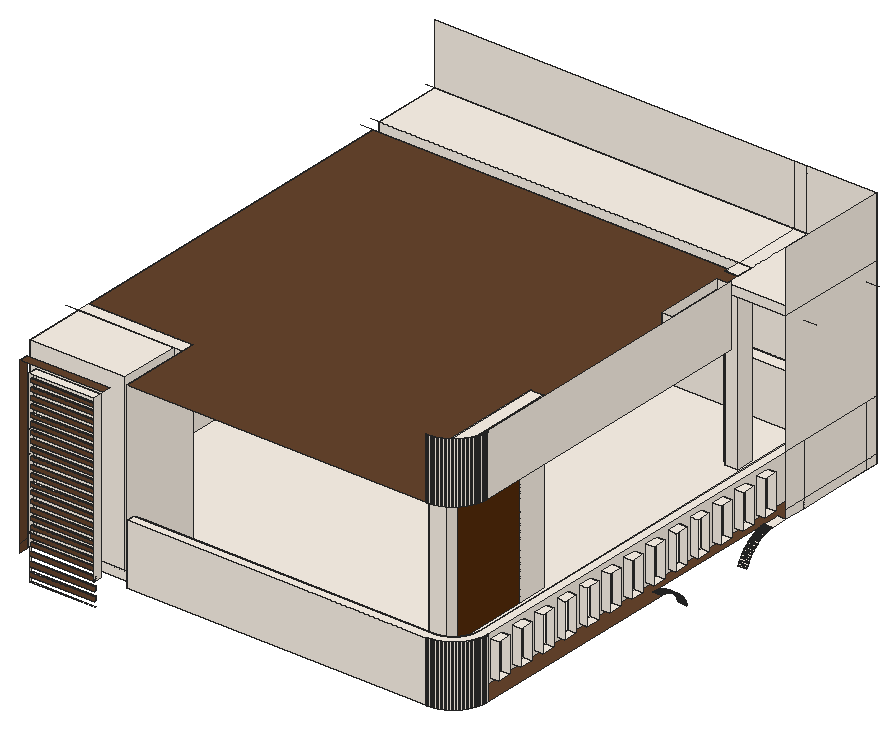
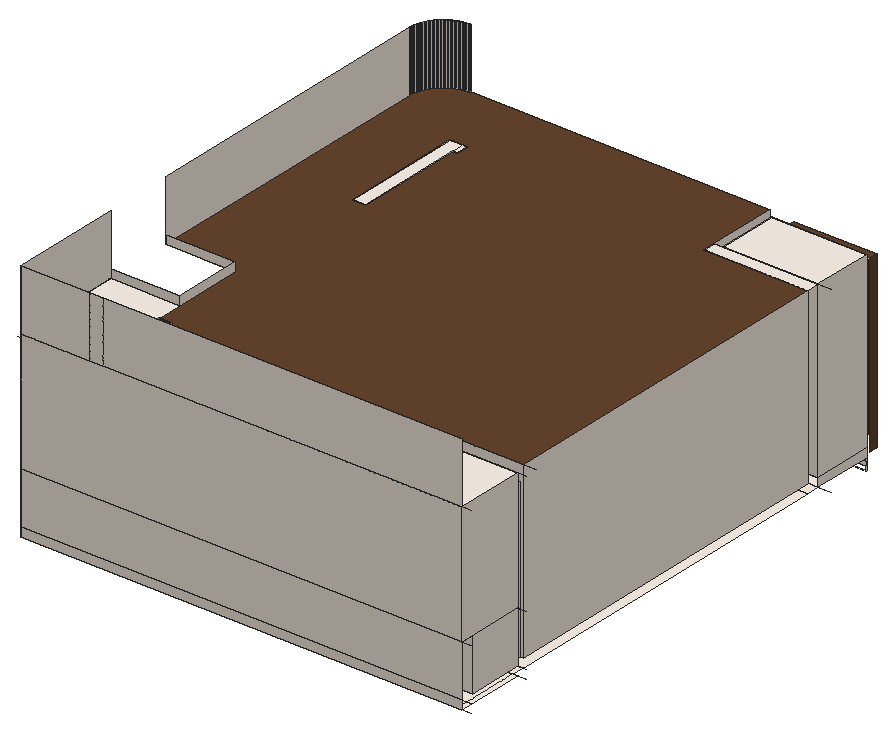
# SketchUp Ruby script. Lengths in inches.
U = 1.inch
M = Sketchup.active_model
def pt(a) = Geom::Point3d.new(a.map { |v| v * U })
def face(e, loops, mat)
  f = e.add_face(loops[0].map { |a| pt(a) })
  loops[1..].each { |l| e.add_face(l.map { |a| pt(a) }).erase! }
  f.material = f.back_material = mat if mat
  f
end
# faces: each face lists its corners as indices into pts; further lists are holes
def faces(e, pts, list, mat = nil) = list.each { |f| face(e, (f[0].is_a?(Array) ? f : [f]).map { |l| l.map { |i| pts[i] } }, mat) }
# xy, xz, yz: faces in a plane at the given z, y or x. An outline is a flat list of corners, or four numbers for a rectangle; further outlines are holes
def ring(l) = l.size == 4 ? [[l[0], l[1]], [l[2], l[1]], [l[2], l[3]], [l[0], l[3]]] : l.each_slice(2).to_a
def flat(e, list, mat, &to3) = list.each { |f| face(e, (f[0].is_a?(Array) ? f : [f]).map { |l| ring(l).map { |u, v| to3.(u, v) } }, mat) }
def xy(e, z, list, mat = nil) = flat(e, list, mat) { |x, y| [x, y, z] }
def xz(e, y, list, mat = nil) = flat(e, list, mat) { |x, z| [x, y, z] }
def yz(e, x, list, mat = nil) = flat(e, list, mat) { |y, z| [x, y, z] }
def lines(e, pts, list) = list.each { |a, b| e.add_line(pt(pts[a]), pt(pts[b])) }
# prism: a flat outline (further loops are holes) pulled along v
def prism(e, loops, v, mat = nil)
  f = face(e, loops, mat); d = Geom::Vector3d.new(v.map { |x| x * U })
  f.pushpull(f.normal.samedirection?(d) ? d.length : -d.length)
end
def box(e, o, s, mat = nil) = prism(e, [[o, [o[0] + s[0], o[1], o[2]], [o[0] + s[0], o[1] + s[1], o[2]], [o[0], o[1] + s[1], o[2]]]], [0, 0, s[2]], mat)
def at(x, y, z, deg = 0) = Geom::Transformation.translation(pt([x, y, z])) * Geom::Transformation.rotation(ORIGIN, Z_AXIS, deg.degrees)
def axes(o, x, y, z) = Geom::Transformation.new([*x, 0, *y, 0, *z, 0, *pt(o).to_a, 1])
def part(name) = M.definitions.add(name)
# library, detail: a bought-in or finely detailed component or shape, given as its bounding box
def library(name, o, s) = part(name).tap { |d| box(d.entities, o, s) }
def detail(e, o, s) = box(e.add_group.entities, o, s)
def put(e, d, t, mat = nil) = e.add_instance(d, t).tap { |i| i.material = mat if mat }
def group(e, t, mat = nil) = e.add_group.tap { |g| g.transformation = t; g.material = mat if mat }.entities
root = M.entities
M.materials.add("C01_Vanilla_Cream").color = [255, 246, 235]
M.materials.add("Earth_Compacted_Fill_1K").color = [86, 45, 11]
M.materials.add("Wood_Veneer_15_1K").color = [103, 69, 45]
xy(root,505.95,[[66,1,111,2]],"C01_Vanilla_Cream")
xy(root,509.1,[[66,1,111,2]],"C01_Vanilla_Cream")
xy(root,512.25,[[66,1,111,2]],"C01_Vanilla_Cream")
xy(root,515.4,[[66,1,111,2]],"C01_Vanilla_Cream")
xy(root,518.55,[[66,1,111,2]],"C01_Vanilla_Cream")
xy(root,521.7,[[66,1,111,2]],"C01_Vanilla_Cream")
xy(root,522,[[57,12,123,54],[123,12,129,54],[57,54,312,63],[57,63,303,309],[303,63,312,309],
  [354,276,360,288],[57,309,312,318],[312,309,360,366],[54,318,57,366],[57,318,312,366]],"C01_Vanilla_Cream")
xy(root,522,[[129,6,129,54,312,54,312,309,360,309,360,288,354,288,354,180,360,180,360,30,359.99,29.25,359.95,28.49,359.89,27.74,359.8125,26.99,359.7,26.25,359.57,25.5,359.42,24.76,359.25,24.03,359.05,23.3,358.83,22.58,358.58,21.87,358.31,21.17,358.03,20.47,357.72,19.78,357.38,19.1,357.03,18.4375,356.66,17.78,356.26,17.14,355.85,16.51,355.42,15.89,354.96,15.29,354.49,14.7,354,14.13,353.5,13.57,352.97,13.03,352.43,12.5,351.87,12,351.3,11.51,350.71,11.04,350.11,10.58,349.49,10.15,348.86,9.74,348.22,9.34,347.5625,8.97,346.9,8.62,346.22,8.28,345.53,7.97,344.83,7.69,344.13,7.42,343.42,7.17,342.7,6.95,341.97,6.75,341.24,6.58,340.5,6.43,339.75,6.3,339.01,6.1875,338.26,6.11,337.51,6.05,336.75,6.01,336,6]],"Wood_Veneer_15_1K")
xy(root,524.85,[[66,1,111,2]],"C01_Vanilla_Cream")
xy(root,528,[[66,1,111,2],[[129,12,336,12,336.57,12.01,337.13,12.04,337.69,12.08,338.26,12.14,338.82,12.22,339.37,12.32,339.93,12.43,340.48,12.57,341.02,12.71,341.5625,12.88,342.1,13.0625,342.625,13.26,343.15,13.48,343.66,13.71,344.17,13.96,344.67,14.23,345.16,14.51,345.64,14.8,346.12,15.11,346.58,15.4375,347.03,15.78,347.47,16.13,347.9,16.5,348.32,16.88,348.73,17.27,349.12,17.68,349.5,18.1,349.87,18.53,350.22,18.97,350.5625,19.42,350.89,19.88,351.2,20.36,351.49,20.84,351.77,21.33,352.04,21.83,352.29,22.34,352.52,22.85,352.74,23.375,352.9375,23.9,353.12,24.4375,353.29,24.98,353.43,25.52,353.57,26.07,353.68,26.63,353.78,27.18,353.86,27.74,353.92,28.31,353.96,28.87,353.99,29.43,354,30,354,357,54,357,54,318,60,318,60,309,57,309,57,63,129,63],[300,54,300,63,303,63,303,138.51,312,138.51,312,54],[303,306,303,309,300,309,300,318,312,318,312,306]],[57,12,123,54],[123,12,129,54],[300,54,300,63,303,63,303,138.51,312,138.51,312,54],
  [303,306,303,309,300,309,300,318,312,318,312,306]],"C01_Vanilla_Cream")
xy(root,530.67,[[66,1,111,2]],"C01_Vanilla_Cream")
xy(root,531,[[354,39,360,48.6],[354,58.2,360,67.8],[354,77.4,360,87],[354,96.6,360,106.2],[354,115.8,360,125.4],
  [354,135,360,144.6],[354,154.2,360,163.8],[354,173.4,360,183],[354,192.6,360,202.2],[354,211.8,360,221.4],
  [354,231,360,240.6],[354,250.2,360,259.8],[354,269.4,360,279]],"C01_Vanilla_Cream")
xy(root,533.35,[[66,1,111,2]],"C01_Vanilla_Cream")
xy(root,536.02,[[66,1,111,2]],"C01_Vanilla_Cream")
xy(root,538.7,[[66,1,111,2]],"C01_Vanilla_Cream")
xy(root,541.375,[[66,1,111,2]],"C01_Vanilla_Cream")
xy(root,544.05,[[66,1,111,2]],"C01_Vanilla_Cream")
xy(root,546.72,[[66,1,111,2]],"C01_Vanilla_Cream")
xy(root,549.4,[[66,1,111,2]],"C01_Vanilla_Cream")
xy(root,552.08,[[66,1,111,2]],"C01_Vanilla_Cream")
xy(root,554.75,[[66,1,111,2]],"C01_Vanilla_Cream")
xy(root,555,[[354,39,360,48.6],[354,58.2,360,67.8],[354,77.4,360,87],[354,96.6,360,106.2],[354,115.8,360,125.4],
  [354,135,360,144.6],[354,154.2,360,163.8],[354,173.4,360,183],[354,192.6,360,202.2],[354,211.8,360,221.4],
  [354,231,360,240.6],[354,250.2,360,259.8],[354,269.4,360,279]],"C01_Vanilla_Cream")
xy(root,557.42,[[66,1,111,2]],"C01_Vanilla_Cream")
xy(root,560.1,[[66,1,111,2]],"C01_Vanilla_Cream")
xy(root,562.78,[[66,1,111,2]],"C01_Vanilla_Cream")
xy(root,564,[[129,6,336,6,336.75,6.01,337.51,6.05,338.26,6.11,339.01,6.1875,339.75,6.3,340.5,6.43,341.24,6.58,341.97,6.75,342.7,6.95,343.42,7.17,344.13,7.42,344.83,7.69,345.53,7.97,346.22,8.28,346.9,8.62,347.5625,8.97,348.22,9.34,348.86,9.74,349.49,10.15,350.11,10.58,350.71,11.04,351.3,11.51,351.87,12,352.43,12.5,352.97,13.03,353.5,13.57,354,14.13,354.49,14.7,354.96,15.29,355.42,15.89,355.85,16.51,356.26,17.14,356.66,17.78,357.03,18.4375,357.38,19.1,357.72,19.78,358.03,20.47,358.31,21.17,358.58,21.87,358.83,22.58,359.05,23.3,359.25,24.03,359.42,24.76,359.57,25.5,359.7,26.25,359.8125,26.99,359.89,27.74,359.95,28.49,359.99,29.25,360,30,360,366,54,366,54,357,354,357,354,30,353.99,29.43,353.96,28.87,353.92,28.31,353.86,27.74,353.78,27.18,353.68,26.63,353.57,26.07,353.43,25.52,353.29,24.98,353.12,24.4375,352.9375,23.9,352.74,23.375,352.52,22.85,352.29,22.34,352.04,21.83,351.77,21.33,351.49,20.84,351.2,20.36,350.89,19.88,350.5625,19.42,350.22,18.97,349.87,18.53,349.5,18.1,349.12,17.68,348.73,17.27,348.32,16.88,347.9,16.5,347.47,16.13,347.03,15.78,346.58,15.4375,346.12,15.11,345.64,14.8,345.16,14.51,344.67,14.23,344.17,13.96,343.66,13.71,343.15,13.48,342.625,13.26,342.1,13.0625,341.5625,12.88,341.02,12.71,340.48,12.57,339.93,12.43,339.37,12.32,338.82,12.22,338.26,12.14,337.69,12.08,337.13,12.04,336.57,12.01,336,12,129,12]],"C01_Vanilla_Cream")
xy(root,565.45,[[66,1,111,2]],"C01_Vanilla_Cream")
xy(root,568.125,[[66,1,111,2]],"C01_Vanilla_Cream")
xy(root,570.8,[[66,1,111,2]],"C01_Vanilla_Cream")
xy(root,573.48,[[66,1,111,2]],"C01_Vanilla_Cream")
xy(root,576.15,[[66,1,111,2]],"C01_Vanilla_Cream")
xy(root,578.82,[[66,1,111,2]],"C01_Vanilla_Cream")
xy(root,581.5,[[66,1,111,2]],"C01_Vanilla_Cream")
xy(root,584.17,[[66,1,111,2]],"C01_Vanilla_Cream")
xy(root,586.85,[[66,1,111,2]],"C01_Vanilla_Cream")
xy(root,589.52,[[66,1,111,2]],"C01_Vanilla_Cream")
xy(root,592.2,[[66,1,111,2]],"C01_Vanilla_Cream")
xy(root,594.875,[[66,1,111,2]],"C01_Vanilla_Cream")
xy(root,597.55,[[66,1,111,2]],"C01_Vanilla_Cream")
xy(root,600.22,[[66,1,111,2]],"C01_Vanilla_Cream")
xy(root,602.9,[[66,1,111,2]],"C01_Vanilla_Cream")
xy(root,605.57,[[66,1,111,2]],"C01_Vanilla_Cream")
xy(root,608.25,[[66,1,111,2]],"C01_Vanilla_Cream")
xy(root,610.92,[[66,1,111,2]],"C01_Vanilla_Cream")
xy(root,613.6,[[66,1,111,2]],"C01_Vanilla_Cream")
xy(root,616.28,[[66,1,111,2]],"C01_Vanilla_Cream")
xy(root,618.95,[[66,1,111,2]],"C01_Vanilla_Cream")
xy(root,621.625,[[66,1,111,2]],"C01_Vanilla_Cream")
xy(root,624.3,[[66,1,111,2]],"C01_Vanilla_Cream")
xy(root,626.97,[[66,1,111,2]],"C01_Vanilla_Cream")
xy(root,629.65,[[66,1,111,2]],"C01_Vanilla_Cream")
xy(root,632.32,[[66,1,111,2]],"C01_Vanilla_Cream")
xy(root,636,[[66,0,111,6],[60,309,300,318]],"C01_Vanilla_Cream")
xy(root,642,[[60,0,117,6]],"Wood_Veneer_15_1K")
xy(root,648,[[57,12,123,54],[57,54,129,63],[300,54,303,63],[303,54,312,138.51],[312,288,360,366],
  [303,306,312,318],[54,318,303,366],[303,318,312,366]],"C01_Vanilla_Cream")
xy(root,648,[[[129,6,129,63,57,63,57,309,303,309,303,306,312,306,312,240,360,240,360,30,359.99,29.25,359.95,28.49,359.89,27.74,359.8125,26.99,359.7,26.25,359.57,25.5,359.42,24.76,359.25,24.03,359.05,23.3,358.83,22.58,358.58,21.87,358.31,21.17,358.03,20.47,357.72,19.78,357.38,19.1,357.03,18.4375,356.66,17.78,356.26,17.14,355.85,16.51,355.42,15.89,354.96,15.29,354.49,14.7,354,14.13,353.5,13.57,352.97,13.03,352.43,12.5,351.87,12,351.3,11.51,350.71,11.04,350.11,10.58,349.49,10.15,348.86,9.74,348.22,9.34,347.5625,8.97,346.9,8.62,346.22,8.28,345.53,7.97,344.83,7.69,344.13,7.42,343.42,7.17,342.7,6.95,341.97,6.75,341.24,6.58,340.5,6.43,339.75,6.3,339.01,6.1875,338.26,6.11,337.51,6.05,336.75,6.01,336,6],[300,54,312,54,312,138.51,303,138.51,303,63,300,63]]],"Wood_Veneer_15_1K")
xz(root,1,[[66,509.1,111,512.25],[66,515.4,111,518.55],[66,521.7,111,524.85],[66,528,111,530.67],[66,533.35,111,536.02],
  [66,538.7,111,541.375],[66,544.05,111,546.72],[66,549.4,111,552.08],[66,554.75,111,557.42],[66,560.1,111,562.78],
  [66,565.45,111,568.125],[66,570.8,111,573.48],[66,576.15,111,578.82],[66,581.5,111,584.17],[66,586.85,111,589.52],
  [66,592.2,111,594.875],[66,597.55,111,600.22],[66,602.9,111,605.57],[66,608.25,111,610.92],[66,613.6,111,616.28],
  [66,618.95,111,621.625],[66,624.3,111,626.97],[66,629.65,111,632.32]],"Wood_Veneer_15_1K")
xz(root,2,[[66,509.1,111,512.25],[66,515.4,111,518.55],[66,521.7,111,524.85],[66,528,111,530.67],[66,533.35,111,536.02],
  [66,538.7,111,541.375],[66,544.05,111,546.72],[66,549.4,111,552.08],[66,554.75,111,557.42],[66,560.1,111,562.78],
  [66,565.45,111,568.125],[66,570.8,111,573.48],[66,576.15,111,578.82],[66,581.5,111,584.17],[66,586.85,111,589.52],
  [66,592.2,111,594.875],[66,597.55,111,600.22],[66,602.9,111,605.57],[66,608.25,111,610.92],[66,613.6,111,616.28],
  [66,618.95,111,621.625],[66,624.3,111,626.97],[66,629.65,111,632.32]],"C01_Vanilla_Cream")
xz(root,6,[[129,522,336,564],[66,528,111,636]],"C01_Vanilla_Cream")
xz(root,12,[[57,522,129,528],[57,528,123,648],[129,528,135,564],[135,528,336,564]],"C01_Vanilla_Cream")
xz(root,39,[[354,531,360,555]],"C01_Vanilla_Cream")
xz(root,48.6,[[354,531,360,555]],"C01_Vanilla_Cream")
xz(root,54,[[57,528,123,648],[300,528,312,648]],"C01_Vanilla_Cream")
xz(root,58.2,[[354,531,360,555]],"C01_Vanilla_Cream")
xz(root,63,[[57,528,129,648],[300,528,303,648]],"C01_Vanilla_Cream")
xz(root,67.8,[[354,531,360,555]],"C01_Vanilla_Cream")
xz(root,77.4,[[354,531,360,555]],"C01_Vanilla_Cream")
xz(root,87,[[354,531,360,555]],"C01_Vanilla_Cream")
xz(root,96.6,[[354,531,360,555]],"C01_Vanilla_Cream")
xz(root,106.2,[[354,531,360,555]],"C01_Vanilla_Cream")
xz(root,115.8,[[354,531,360,555]],"C01_Vanilla_Cream")
xz(root,125.4,[[354,531,360,555]],"C01_Vanilla_Cream")
xz(root,135,[[354,531,360,555]],"C01_Vanilla_Cream")
xz(root,138.51,[[303,528,312,648]],"C01_Vanilla_Cream")
xz(root,144.6,[[354,531,360,555]],"C01_Vanilla_Cream")
xz(root,154.2,[[354,531,360,555]],"C01_Vanilla_Cream")
xz(root,163.8,[[354,531,360,555]],"C01_Vanilla_Cream")
xz(root,173.4,[[354,531,360,555]],"C01_Vanilla_Cream")
xz(root,183,[[354,531,360,555]],"C01_Vanilla_Cream")
xz(root,192.6,[[354,531,360,555]],"C01_Vanilla_Cream")
xz(root,202.2,[[354,531,360,555]],"C01_Vanilla_Cream")
xz(root,211.8,[[354,531,360,555]],"C01_Vanilla_Cream")
xz(root,221.4,[[354,531,360,555]],"C01_Vanilla_Cream")
xz(root,231,[[354,531,360,555]],"C01_Vanilla_Cream")
xz(root,240,[[312,648,360,654]],"C01_Vanilla_Cream")
xz(root,240.6,[[354,531,360,555]],"C01_Vanilla_Cream")
xz(root,250.2,[[354,531,360,555]],"C01_Vanilla_Cream")
xz(root,259.8,[[354,531,360,555]],"C01_Vanilla_Cream")
xz(root,269.4,[[354,531,360,555]],"C01_Vanilla_Cream")
xz(root,279,[[354,531,360,555]],"C01_Vanilla_Cream")
xz(root,288,[[312,648,360,654]],"C01_Vanilla_Cream")
xz(root,306,[[303,528,312,648]],"C01_Vanilla_Cream")
xz(root,309,[[57,528,60,528,60,636,300,636,300,528,303,528,303,648,57,648]],"C01_Vanilla_Cream")
xz(root,318,[[54,528,54,648,312,648,312,528,300,528,300,636,60,636,60,528]],"C01_Vanilla_Cream")
xz(root,357,[[54,528,354,564]],"C01_Vanilla_Cream")
xz(root,366,[[54,522,360,528],[54,528,360,564],[54,564,360,648],[54,648,303,690],[303,648,312,690],
  [312,648,360,690]],"C01_Vanilla_Cream")
yz(root,54,[[318,528,357,564],[318,564,366,648]],"C01_Vanilla_Cream")
yz(root,57,[[12,522,54,528],[12,528,54,648],[63,528,309,648]],"C01_Vanilla_Cream")
yz(root,60,[[309,528,318,636]],"C01_Vanilla_Cream")
yz(root,60,[[0,522,6,528],[0,528,6,642]],"Wood_Veneer_15_1K")
yz(root,66,[[1,505.95,2,509.1],[1,512.25,2,515.4],[1,518.55,2,521.7],[1,524.85,2,528],[0,528,1,528,1,635,2,635,2,528,3,528,3,636,0,636],
  [3,528,6,636],[1,530.67,2,533.35],[1,536.02,2,538.7],[1,541.375,2,544.05],[1,546.72,2,549.4],
  [1,552.08,2,554.75],[1,557.42,2,560.1],[1,562.78,2,565.45],[1,568.125,2,570.8],[1,573.48,2,576.15],
  [1,578.82,2,581.5],[1,584.17,2,586.85],[1,589.52,2,592.2],[1,594.875,2,597.55],[1,600.22,2,602.9],
  [1,605.57,2,608.25],[1,610.92,2,613.6],[1,616.28,2,618.95],[1,621.625,2,624.3],[1,626.97,2,629.65],
  [1,632.32,2,635]],"C01_Vanilla_Cream")
yz(root,111,[[1,521.7,2,522],[[0,522,0,636,6,636,6,522,2,522,2,524.85,1,524.85,1,522],[1,544.05,2,546.72],[1,549.4,2,552.08],[1,570.8,2,573.48],[1,592.2,2,594.875],[1,613.6,2,616.28],[1,618.95,2,621.625],[1,528,2,530.67],[1,533.35,2,536.02],[1,538.7,2,541.375],[1,554.75,2,557.42],[1,560.1,2,562.78],[1,565.45,2,568.125],[1,576.15,2,578.82],[1,581.5,2,584.17],[1,586.85,2,589.52],[1,597.55,2,600.22],[1,602.9,2,605.57],[1,608.25,2,610.92],[1,624.3,2,626.97],[1,629.65,2,632.32]],[1,522,2,524.85]],"C01_Vanilla_Cream")
yz(root,123,[[12,528,54,648]],"C01_Vanilla_Cream")
yz(root,129,[[6,522,12,528],[12,528,63,528,63,648,6,648,6,564,12,564],[6,528,12,564]],"C01_Vanilla_Cream")
yz(root,300,[[54,528,63,648],[309,528,318,636]],"C01_Vanilla_Cream")
yz(root,303,[[63,528,138.51,648],[306,528,309,648]],"C01_Vanilla_Cream")
yz(root,312,[[54,528,63,648],[117,528,138.51,648],[306,528,318,648],[240,648,288,654]],"C01_Vanilla_Cream")
yz(root,312,[[63,528,117,648]],"Earth_Compacted_Fill_1K")
yz(root,354,[[[30,528,357,564],[269.4,531,279,555],[250.2,531,259.8,555],[192.6,531,202.2,555],[115.8,531,125.4,555],[96.6,531,106.2,555],[231,531,240.6,555],[211.8,531,221.4,555],[173.4,531,183,555],[154.2,531,163.8,555],[135,531,144.6,555],[77.4,531,87,555],[58.2,531,67.8,555],[39,531,48.6,555]]],"C01_Vanilla_Cream")
yz(root,360,[[288,522,303,528],[303,522,357,528],[357,522,366,528],[288,528,303,564],[303,528,357,564],
  [357,528,366,564],[288,564,366,648],[30,648,240,690],[288,648,366,690]],"C01_Vanilla_Cream")
p = [[360,254.25,506.5],[360,253.95,505.83],[354,253.95,505.83],[354,254.25,506.5],[360,202.36,506.01],[360,202.09,506.7],
  [354,202.09,506.7],[354,202.36,506.01],[360,254.56,507.17],[354,254.56,507.17],[360,201.79,507.39],[354,201.79,507.39],
  [360,254.89,507.83],[354,254.89,507.83],[360,201.47,508.0625],[354,201.47,508.0625],[360,255.24,508.48],[354,255.24,508.48],
  [360,201.13,508.73],[354,201.13,508.73],[360,255.61,509.12],[354,255.61,509.12],[360,200.77,509.38],[354,200.77,509.38],
  [360,255.99,509.74],[354,255.99,509.74],[360,200.39,510.03],[354,200.39,510.03],[360,256.39,510.36],[354,256.39,510.36],
  [360,200,510.66],[354,200,510.66],[360,256.8125,510.97],[354,256.8125,510.97],[360,199.58,511.28],[354,199.58,511.28],
  [360,257.25,511.56],[354,257.25,511.56],[360,199.15,511.89],[354,199.15,511.89],[360,257.7,512.14],[354,257.7,512.14],
  [360,198.69,512.48],[354,198.69,512.48],[360,258.17,512.71],[354,258.17,512.71],[360,198.22,513.0625],[354,198.22,513.0625],
  [360,258.65,513.27],[354,258.65,513.27],[360,197.74,513.625],[354,197.74,513.625],[360,259.15,513.81],[354,259.15,513.81],
  [360,197.23,514.18],[354,197.23,514.18],[360,259.66,514.34],[354,259.66,514.34],[360,196.71,514.71],[354,196.71,514.71],
  [360,260.19,514.85],[354,260.19,514.85],[360,196.18,515.23],[354,196.18,515.23],[360,260.73,515.35],[354,260.73,515.35],
  [360,195.625,515.74],[354,195.625,515.74],[360,261.29,515.83],[354,261.29,515.83],[360,195.0625,516.22],[354,195.0625,516.22],
  [360,261.86,516.3],[354,261.86,516.3],[360,194.48,516.69],[354,194.48,516.69],[360,262.44,516.75],[354,262.44,516.75],
  [360,193.89,517.15],[354,193.89,517.15],[360,263.03,517.1875],[354,263.03,517.1875],[360,193.28,517.58],[354,193.28,517.58],
  [360,263.64,517.61],[354,263.64,517.61],[360,192.66,518],[354,192.66,518],[360,264.26,518.01],[354,264.26,518.01],
  [360,192.03,518.39],[354,192.03,518.39],[360,264.88,518.39],[354,264.88,518.39],[360,191.38,518.77],[354,191.38,518.77],
  [360,265.52,518.76],[354,265.52,518.76],[360,190.73,519.13],[354,190.73,519.13],[360,266.17,519.11],[354,266.17,519.11],
  [360,190.0625,519.47],[354,190.0625,519.47],[360,266.83,519.44],[354,266.83,519.44],[360,267.5,519.75],[354,267.5,519.75],
  [360,189.39,519.79],[354,189.39,519.79],[360,188.7,520.09],[354,188.7,520.09],[360,268.17,520.05],[354,268.17,520.05],
  [360,268.85,520.32],[354,268.85,520.32],[360,188.01,520.36],[354,188.01,520.36],[360,269.54,520.58],[354,269.54,520.58],
  [360,187.31,520.62],[354,187.31,520.62],[360,186.6,520.86],[354,186.6,520.86],[360,270.24,520.82],[354,270.24,520.82],
  [360,270.94,521.03],[354,270.94,521.03],[360,185.89,521.07],[354,185.89,521.07],[360,271.65,521.23],[354,271.65,521.23],
  [360,185.16,521.26],[354,185.16,521.26],[360,272.37,521.41],[354,272.37,521.41],[360,184.4375,521.44],[354,184.4375,521.44],
  [360,183.71,521.58],[354,183.71,521.58],[360,273.09,521.57],[354,273.09,521.57],[360,182.97,521.71],[354,182.97,521.71],
  [360,273.8125,521.71],[354,273.8125,521.71],[360,182.23,521.82],[354,182.23,521.82],[360,274.54,521.82],[354,274.54,521.82],
  [360,181.49,521.9],[354,181.49,521.9],[360,275.27,521.92],[354,275.27,521.92],[360,180.75,521.96],[354,180.75,521.96],
  [360,276,522],[354,276,522],[336.75,6.01,522],[336.75,6.01,564],[336,6,564],[336,6,522],
  [337.51,6.05,522],[337.51,6.05,564],[338.26,6.11,522],[338.26,6.11,564],[339.01,6.1875,522],[339.01,6.1875,564],
  [339.75,6.3,522],[339.75,6.3,564],[340.5,6.43,522],[340.5,6.43,564],[341.24,6.58,522],[341.24,6.58,564],
  [341.97,6.75,522],[341.97,6.75,564],[342.7,6.95,522],[342.7,6.95,564],[343.42,7.17,522],[343.42,7.17,564],
  [344.13,7.42,522],[344.13,7.42,564],[344.83,7.69,522],[344.83,7.69,564],[345.53,7.97,522],[345.53,7.97,564],
  [346.22,8.28,522],[346.22,8.28,564],[346.9,8.62,522],[346.9,8.62,564],[347.5625,8.97,522],[347.5625,8.97,564],
  [348.22,9.34,522],[348.22,9.34,564],[348.86,9.74,522],[348.86,9.74,564],[349.49,10.15,522],[349.49,10.15,564],
  [350.11,10.58,522],[350.11,10.58,564],[350.71,11.04,522],[350.71,11.04,564],[351.3,11.51,522],[351.3,11.51,564],
  [351.87,12,522],[351.87,12,564],[352.43,12.5,522],[352.43,12.5,564],[352.97,13.03,522],[352.97,13.03,564],
  [353.5,13.57,522],[353.5,13.57,564],[354,14.13,522],[354,14.13,564],[354.49,14.7,522],[354.49,14.7,564],
  [354.96,15.29,522],[354.96,15.29,564],[355.42,15.89,522],[355.42,15.89,564],[355.85,16.51,522],[355.85,16.51,564],
  [356.26,17.14,522],[356.26,17.14,564],[356.66,17.78,522],[356.66,17.78,564],[357.03,18.4375,522],[357.03,18.4375,564],
  [357.38,19.1,522],[357.38,19.1,564],[357.72,19.78,522],[357.72,19.78,564],[358.03,20.47,522],[358.03,20.47,564],
  [358.31,21.17,522],[358.31,21.17,564],[358.58,21.87,522],[358.58,21.87,564],[358.83,22.58,522],[358.83,22.58,564],
  [359.05,23.3,522],[359.05,23.3,564],[359.25,24.03,522],[359.25,24.03,564],[359.42,24.76,522],[359.42,24.76,564],
  [359.57,25.5,522],[359.57,25.5,564],[359.7,26.25,522],[359.7,26.25,564],[359.8125,26.99,522],[359.8125,26.99,564],
  [359.89,27.74,522],[359.89,27.74,564],[359.95,28.49,522],[359.95,28.49,564],[359.99,29.25,522],[359.99,29.25,564],
  [360,30,522],[360,30,564],[360,180,522],[354,180,522],[336.57,12.01,528],[336,12,528],
  [336,12,564],[336.57,12.01,564],[337.13,12.04,528],[337.13,12.04,564],[337.69,12.08,528],[337.69,12.08,564],
  [338.26,12.14,528],[338.26,12.14,564],[338.82,12.22,528],[338.82,12.22,564],[339.37,12.32,528],[339.37,12.32,564],
  [339.93,12.43,528],[339.93,12.43,564],[340.48,12.57,528],[340.48,12.57,564],[341.02,12.71,528],[341.02,12.71,564],
  [341.5625,12.88,528],[341.5625,12.88,564],[342.1,13.0625,528],[342.1,13.0625,564],[342.625,13.26,528],[342.625,13.26,564],
  [343.15,13.48,528],[343.15,13.48,564],[343.66,13.71,528],[343.66,13.71,564],[344.17,13.96,528],[344.17,13.96,564],
  [344.67,14.23,528],[344.67,14.23,564],[345.16,14.51,528],[345.16,14.51,564],[345.64,14.8,528],[345.64,14.8,564],
  [346.12,15.11,528],[346.12,15.11,564],[346.58,15.4375,528],[346.58,15.4375,564],[347.03,15.78,528],[347.03,15.78,564],
  [347.47,16.13,528],[347.47,16.13,564],[347.9,16.5,528],[347.9,16.5,564],[348.32,16.88,528],[348.32,16.88,564],
  [348.73,17.27,528],[348.73,17.27,564],[349.12,17.68,528],[349.12,17.68,564],[349.5,18.1,528],[349.5,18.1,564],
  [349.87,18.53,528],[349.87,18.53,564],[350.22,18.97,528],[350.22,18.97,564],[350.5625,19.42,528],[350.5625,19.42,564],
  [350.89,19.88,528],[350.89,19.88,564],[351.2,20.36,528],[351.2,20.36,564],[351.49,20.84,528],[351.49,20.84,564],
  [351.77,21.33,528],[351.77,21.33,564],[352.04,21.83,528],[352.04,21.83,564],[352.29,22.34,528],[352.29,22.34,564],
  [352.52,22.85,528],[352.52,22.85,564],[352.74,23.375,528],[352.74,23.375,564],[352.9375,23.9,528],[352.9375,23.9,564],
  [353.12,24.4375,528],[353.12,24.4375,564],[353.29,24.98,528],[353.29,24.98,564],[353.43,25.52,528],[353.43,25.52,564],
  [353.57,26.07,528],[353.57,26.07,564],[353.68,26.63,528],[353.68,26.63,564],[353.78,27.18,528],[353.78,27.18,564],
  [353.86,27.74,528],[353.86,27.74,564],[353.92,28.31,528],[353.92,28.31,564],[353.96,28.87,528],[353.96,28.87,564],
  [353.99,29.43,528],[353.99,29.43,564],[354,30,528],[354,30,564],[336.75,6.01,648],[336.75,6.01,690],
  [336,6,690],[336,6,648],[337.51,6.05,648],[337.51,6.05,690],[338.26,6.11,648],[338.26,6.11,690],
  [339.01,6.1875,648],[339.01,6.1875,690],[339.75,6.3,648],[339.75,6.3,690],[340.5,6.43,648],[340.5,6.43,690],
  [341.24,6.58,648],[341.24,6.58,690],[341.97,6.75,648],[341.97,6.75,690],[342.7,6.95,648],[342.7,6.95,690],
  [343.42,7.17,648],[343.42,7.17,690],[344.13,7.42,648],[344.13,7.42,690],[344.83,7.69,648],[344.83,7.69,690],
  [345.53,7.97,648],[345.53,7.97,690],[346.22,8.28,648],[346.22,8.28,690],[346.9,8.62,648],[346.9,8.62,690],
  [347.5625,8.97,648],[347.5625,8.97,690],[348.22,9.34,648],[348.22,9.34,690],[348.86,9.74,648],[348.86,9.74,690],
  [349.49,10.15,648],[349.49,10.15,690],[350.11,10.58,648],[350.11,10.58,690],[350.71,11.04,648],[350.71,11.04,690],
  [351.3,11.51,648],[351.3,11.51,690],[351.87,12,648],[351.87,12,690],[352.43,12.5,648],[352.43,12.5,690],
  [352.97,13.03,648],[352.97,13.03,690],[353.5,13.57,648],[353.5,13.57,690],[354,14.13,648],[354,14.13,690],
  [354.49,14.7,648],[354.49,14.7,690],[354.96,15.29,648],[354.96,15.29,690],[355.42,15.89,648],[355.42,15.89,690],
  [355.85,16.51,648],[355.85,16.51,690],[356.26,17.14,648],[356.26,17.14,690],[356.66,17.78,648],[356.66,17.78,690],
  [357.03,18.4375,648],[357.03,18.4375,690],[357.38,19.1,648],[357.38,19.1,690],[357.72,19.78,648],[357.72,19.78,690],
  [358.03,20.47,648],[358.03,20.47,690],[358.31,21.17,648],[358.31,21.17,690],[358.58,21.87,648],[358.58,21.87,690],
  [358.83,22.58,648],[358.83,22.58,690],[359.05,23.3,648],[359.05,23.3,690],[359.25,24.03,648],[359.25,24.03,690],
  [359.42,24.76,648],[359.42,24.76,690],[359.57,25.5,648],[359.57,25.5,690],[359.7,26.25,648],[359.7,26.25,690],
  [359.8125,26.99,648],[359.8125,26.99,690],[359.89,27.74,648],[359.89,27.74,690],[359.95,28.49,648],[359.95,28.49,690],
  [359.99,29.25,648],[359.99,29.25,690],[360,30,648],[360,30,690],[48,318,522],[54,318,522],
  [48,54,648],[57,54,648],[57,309,648],[48,309,648],[369,303,639],[360,303,639],
  [369,357,639],[360,357,639],[57,54,522],[48,54,522],[54,318,528],[48,318,528],
  [54,366,648],[48,366,648],[54,366,528],[48,366,528],[54,366,564],[48,366,564],
  [54,366,522],[48,366,522],[54,318,564],[48,318,564],[54,318,648],[48,318,648]]
faces(root,p,[[0,1,2,3],[4,5,6,7],[8,0,3,9],[5,10,11,6],[12,8,9,13],[10,14,15,11],[16,12,13,17],[14,18,19,15],
  [20,16,17,21],[18,22,23,19],[24,20,21,25],[22,26,27,23],[28,24,25,29],[26,30,31,27],[32,28,29,33],[30,34,35,31],
  [36,32,33,37],[34,38,39,35],[40,36,37,41],[38,42,43,39],[44,40,41,45],[42,46,47,43],[48,44,45,49],[46,50,51,47],
  [52,48,49,53],[50,54,55,51],[56,52,53,57],[54,58,59,55],[60,56,57,61],[58,62,63,59],[64,60,61,65],[62,66,67,63],
  [68,64,65,69],[66,70,71,67],[72,68,69,73],[70,74,75,71],[76,72,73,77],[74,78,79,75],[80,76,77,81],[78,82,83,79],
  [84,80,81,85],[82,86,87,83],[88,84,85,89],[86,90,91,87],[92,88,89,93],[90,94,95,91],[96,92,93,97],[94,98,99,95],
  [100,96,97,101],[98,102,103,99],[104,100,101,105],[106,104,105,107],[102,108,109,103],[108,110,111,109],[112,106,107,113],[114,112,113,115],
  [110,116,117,111],[118,114,115,119],[116,120,121,117],[120,122,123,121],[124,118,119,125],[126,124,125,127],[122,128,129,123],[130,126,127,131],
  [128,132,133,129],[134,130,131,135],[132,136,137,133],[136,138,139,137],[140,134,135,141],[138,142,143,139],[144,140,141,145],[142,146,147,143],
  [148,144,145,149],[146,150,151,147],[152,148,149,153],[150,154,155,151],[156,152,153,157],[158,159,160,161],[162,163,159,158],[164,165,163,162],
  [166,167,165,164],[168,169,167,166],[170,171,169,168],[172,173,171,170],[174,175,173,172],[176,177,175,174],[178,179,177,176],[180,181,179,178],
  [182,183,181,180],[184,185,183,182],[186,187,185,184],[188,189,187,186],[190,191,189,188],[192,193,191,190],[194,195,193,192],[196,197,195,194],
  [198,199,197,196],[200,201,199,198],[202,203,201,200],[204,205,203,202],[206,207,205,204],[208,209,207,206],[210,211,209,208],[212,213,211,210],
  [214,215,213,212],[216,217,215,214],[218,219,217,216],[220,221,219,218],[222,223,221,220],[224,225,223,222],[226,227,225,224],[228,229,227,226],
  [230,231,229,228],[232,233,231,230],[234,235,233,232],[236,237,235,234],[238,239,237,236],[240,241,239,238],[242,243,241,240],[244,245,243,242],
  [246,247,245,244],[248,249,247,246],[250,251,249,248],[252,253,251,250],[254,255,253,252],[256,257,255,254],[258,259,257,256],[154,260,261,155],
  [262,263,264,265],[266,262,265,267],[268,266,267,269],[270,268,269,271],[272,270,271,273],[274,272,273,275],[276,274,275,277],[278,276,277,279],
  [280,278,279,281],[282,280,281,283],[284,282,283,285],[286,284,285,287],[288,286,287,289],[290,288,289,291],[292,290,291,293],[294,292,293,295],
  [296,294,295,297],[298,296,297,299],[300,298,299,301],[302,300,301,303],[304,302,303,305],[306,304,305,307],[308,306,307,309],[310,308,309,311],
  [312,310,311,313],[314,312,313,315],[316,314,315,317],[318,316,317,319],[320,318,319,321],[322,320,321,323],[324,322,323,325],[326,324,325,327],
  [328,326,327,329],[330,328,329,331],[332,330,331,333],[334,332,333,335],[336,334,335,337],[338,336,337,339],[340,338,339,341],[342,340,341,343],
  [344,342,343,345],[346,344,345,347],[348,346,347,349],[350,348,349,351],[352,350,351,353],[354,352,353,355],[356,354,355,357],[358,356,357,359],
  [360,358,359,361],[362,360,361,363],[364,365,366,367],[368,369,365,364],[370,371,369,368],[372,373,371,370],[374,375,373,372],[376,377,375,374],
  [378,379,377,376],[380,381,379,378],[382,383,381,380],[384,385,383,382],[386,387,385,384],[388,389,387,386],[390,391,389,388],[392,393,391,390],
  [394,395,393,392],[396,397,395,394],[398,399,397,396],[400,401,399,398],[402,403,401,400],[404,405,403,402],[406,407,405,404],[408,409,407,406],
  [410,411,409,408],[412,413,411,410],[414,415,413,412],[416,417,415,414],[418,419,417,416],[420,421,419,418],[422,423,421,420],[424,425,423,422],
  [426,427,425,424],[428,429,427,426],[430,431,429,428],[432,433,431,430],[434,435,433,432],[436,437,435,434],[438,439,437,436],[440,441,439,438],
  [442,443,441,440],[444,445,443,442],[446,447,445,444],[448,449,447,446],[450,451,449,448],[452,453,451,450],[454,455,453,452],[456,457,455,454],
  [458,459,457,456],[460,461,459,458],[462,463,461,460],[464,465,463,462]],"C01_Vanilla_Cream")
lines(root,p,[[466,467],[468,469],[470,471],[472,473],[474,475],[476,477],[478,479],[480,481],[482,483],[484,485],[486,487],[488,489],
  [490,491]])
